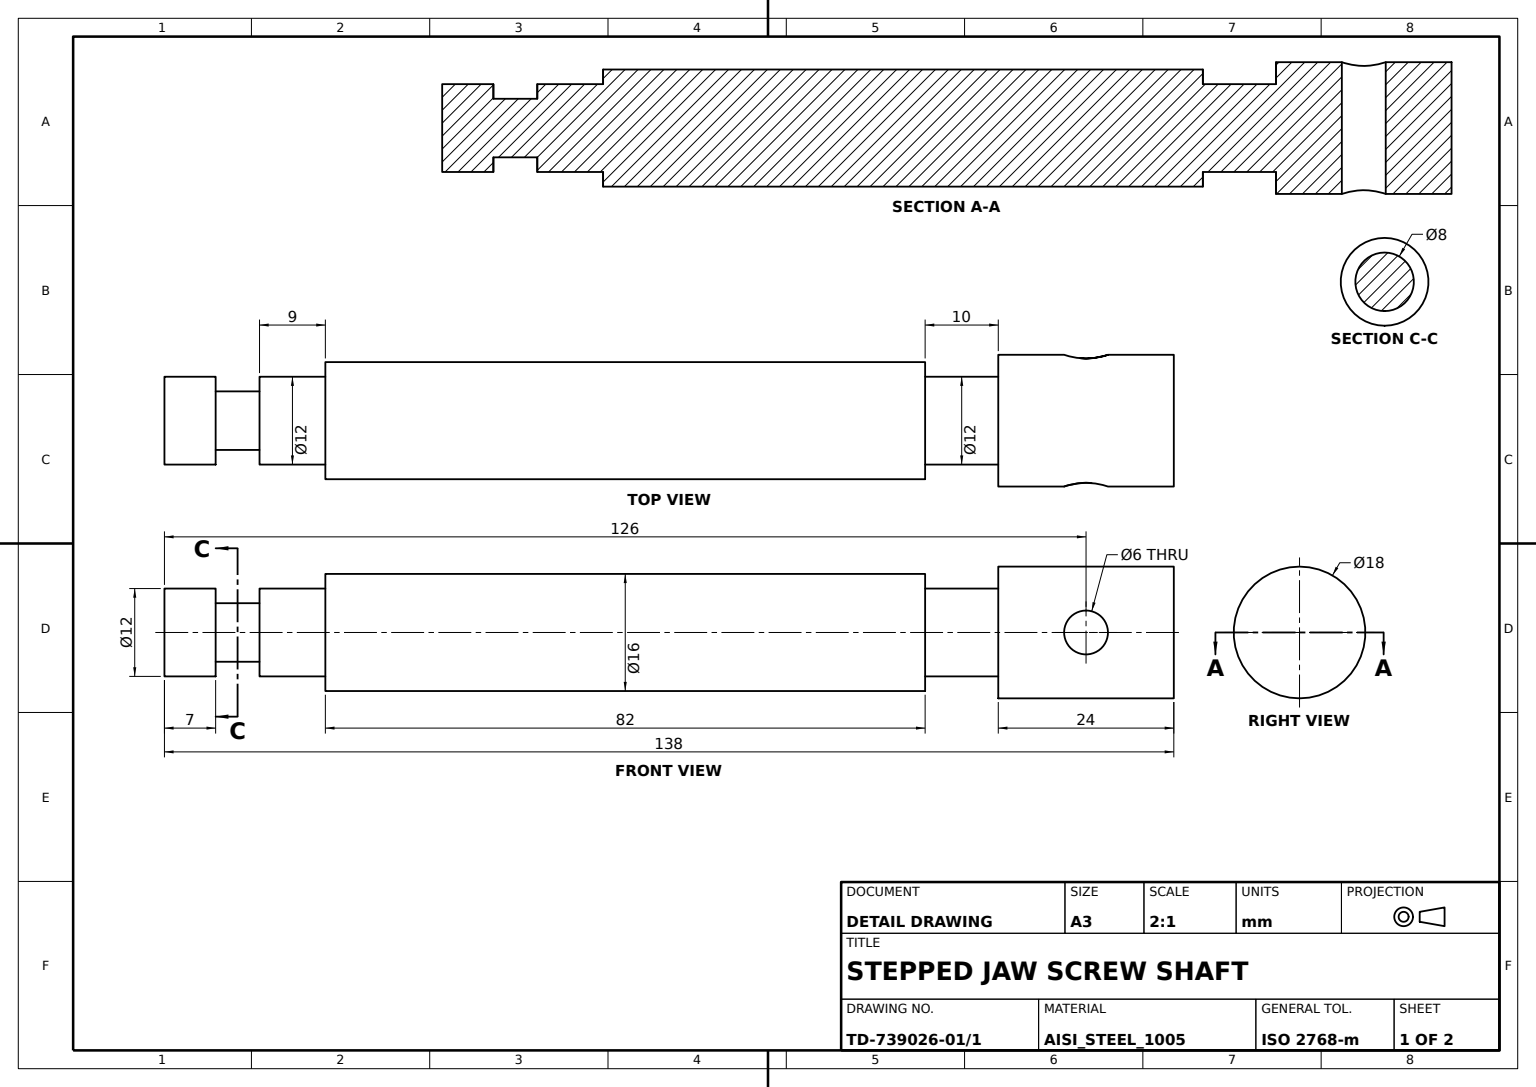
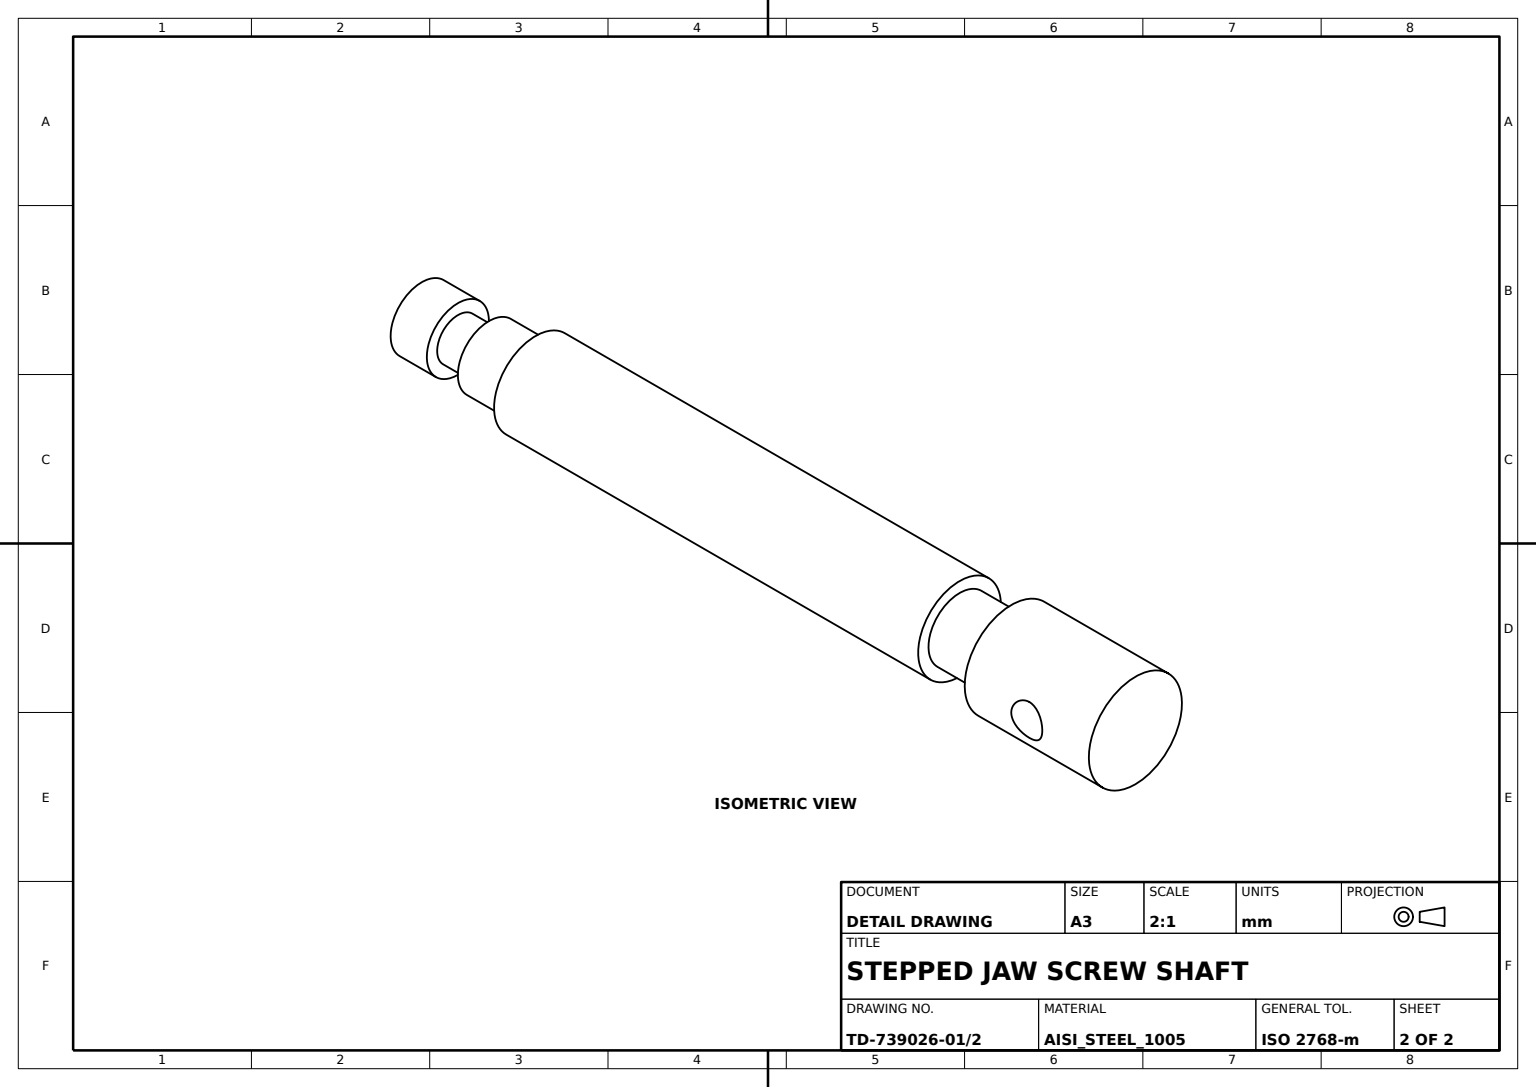
ISO-10303-21;
HEADER;
FILE_DESCRIPTION((''),'2;1');
FILE_NAME('','',(''),(''),'','','');
FILE_SCHEMA(('AUTOMOTIVE_DESIGN'));
ENDSEC;
DATA;
#1=APPLICATION_CONTEXT('');
#2=PRODUCT_CONTEXT('',#1,'mechanical');
#3=PRODUCT('','','',(#2));
#4=PRODUCT_DEFINITION_FORMATION('','',#3);
#5=PRODUCT_DEFINITION_CONTEXT('',#1,'design');
#6=PRODUCT_DEFINITION('','',#4,#5);
#7=PRODUCT_DEFINITION_SHAPE('','',#6);
#8=(LENGTH_UNIT()NAMED_UNIT(*)SI_UNIT(.MILLI.,.METRE.));
#9=(NAMED_UNIT(*)PLANE_ANGLE_UNIT()SI_UNIT($,.RADIAN.));
#10=(NAMED_UNIT(*)SI_UNIT($,.STERADIAN.)SOLID_ANGLE_UNIT());
#11=UNCERTAINTY_MEASURE_WITH_UNIT(LENGTH_MEASURE(0.005),#8,'distance_accuracy_value','');
#12=(GEOMETRIC_REPRESENTATION_CONTEXT(3)GLOBAL_UNCERTAINTY_ASSIGNED_CONTEXT((#11))GLOBAL_UNIT_ASSIGNED_CONTEXT((#8,#9,#10))REPRESENTATION_CONTEXT('',''));
#13=CARTESIAN_POINT('',(0.,48.513563,-9.));
#14=VERTEX_POINT('',#13);
#15=CARTESIAN_POINT('',(0.,48.513563,0.));
#16=DIRECTION('',(0.,-1.,0.));
#17=DIRECTION('',(0.,0.,-1.));
#18=AXIS2_PLACEMENT_3D('',#15,#16,#17);
#19=CIRCLE('',#18,9.);
#20=EDGE_CURVE('',#14,#14,#19,.T.);
#21=ORIENTED_EDGE('',*,*,#20,.T.);
#22=EDGE_LOOP('',(#21));
#23=FACE_BOUND('',#22,.T.);
#24=CARTESIAN_POINT('',(-8.485281,36.513563,3.));
#25=VERTEX_POINT('',#24);
#26=CARTESIAN_POINT('',(-8.75019,34.162799,2.350721));
#27=CARTESIAN_POINT('',(-8.35281,36.513505,3.324938));
#28=CARTESIAN_POINT('',(-8.750258,38.864559,2.349527));
#29=CARTESIAN_POINT('',(-9.124964,39.838536,0.003896));
#30=CARTESIAN_POINT('',(-8.749886,38.862669,-2.353151));
#31=CARTESIAN_POINT('',(-8.352987,36.515667,-3.323633));
#32=CARTESIAN_POINT('',(-8.749854,34.163464,-2.352315));
#33=CARTESIAN_POINT('',(-9.124989,33.188778,0.000128));
#34=B_SPLINE_CURVE_WITH_KNOTS('',3,(#26,#27,#28,#29,#30,#31,#32,#33,#26,#27,#28),.UNSPECIFIED.,.T.,.F.,(1,1,1,1,1,1,1,1,1,1,1,1,1,1,1),(-0.007084493,-0.004722996,-0.002361498,0.,0.002361498,0.004722996,0.007084493,0.009445991,0.011807489,0.014168987,0.016530485,0.018891983,0.02125348,0.023614978,0.025976476),.UNSPECIFIED.);
#35=EDGE_CURVE('',#25,#25,#34,.T.);
#36=ORIENTED_EDGE('',*,*,#35,.F.);
#37=EDGE_LOOP('',(#36));
#38=FACE_BOUND('',#37,.T.);
#39=CARTESIAN_POINT('',(8.485281,36.513563,3.));
#40=VERTEX_POINT('',#39);
#41=CARTESIAN_POINT('',(8.75019,38.864326,2.350721));
#42=CARTESIAN_POINT('',(8.35281,36.513621,3.324938));
#43=CARTESIAN_POINT('',(8.750258,34.162567,2.349527));
#44=CARTESIAN_POINT('',(9.124964,33.188589,0.003896));
#45=CARTESIAN_POINT('',(8.749886,34.164457,-2.353151));
#46=CARTESIAN_POINT('',(8.352987,36.511459,-3.323633));
#47=CARTESIAN_POINT('',(8.749854,38.863662,-2.352315));
#48=CARTESIAN_POINT('',(9.124989,39.838347,0.000128));
#49=B_SPLINE_CURVE_WITH_KNOTS('',3,(#41,#42,#43,#44,#45,#46,#47,#48,#41,#42,#43),.UNSPECIFIED.,.T.,.F.,(1,1,1,1,1,1,1,1,1,1,1,1,1,1,1),(-0.007084493,-0.004722996,-0.002361498,0.,0.002361498,0.004722996,0.007084493,0.009445991,0.011807489,0.014168987,0.016530485,0.018891983,0.02125348,0.023614978,0.025976476),.UNSPECIFIED.);
#50=EDGE_CURVE('',#40,#40,#49,.T.);
#51=ORIENTED_EDGE('',*,*,#50,.F.);
#52=EDGE_LOOP('',(#51));
#53=FACE_BOUND('',#52,.T.);
#54=CARTESIAN_POINT('',(0.,24.513563,-9.));
#55=VERTEX_POINT('',#54);
#56=CARTESIAN_POINT('',(0.,24.513563,0.));
#57=AXIS2_PLACEMENT_3D('',#56,#16,#17);
#58=CIRCLE('',#57,9.);
#59=EDGE_CURVE('',#55,#55,#58,.T.);
#60=ORIENTED_EDGE('',*,*,#59,.F.);
#61=EDGE_LOOP('',(#60));
#62=FACE_BOUND('',#61,.T.);
#63=CARTESIAN_POINT('',(0.,0.,0.));
#64=AXIS2_PLACEMENT_3D('',#63,#16,#17);
#65=CYLINDRICAL_SURFACE('',#64,9.);
#66=ADVANCED_FACE('',(#23,#38,#53,#62),#65,.T.);
#67=CARTESIAN_POINT('',(0.,-67.486437,-8.));
#68=VERTEX_POINT('',#67);
#69=CARTESIAN_POINT('',(0.,-67.486437,0.));
#70=AXIS2_PLACEMENT_3D('',#69,#16,#17);
#71=CIRCLE('',#70,8.);
#72=EDGE_CURVE('',#68,#68,#71,.T.);
#73=ORIENTED_EDGE('',*,*,#72,.T.);
#74=EDGE_LOOP('',(#73));
#75=FACE_BOUND('',#74,.T.);
#76=CARTESIAN_POINT('',(0.,-67.486437,-6.));
#77=VERTEX_POINT('',#76);
#78=CIRCLE('',#70,6.);
#79=EDGE_CURVE('',#77,#77,#78,.T.);
#80=ORIENTED_EDGE('',*,*,#79,.F.);
#81=EDGE_LOOP('',(#80));
#82=FACE_BOUND('',#81,.T.);
#83=CARTESIAN_POINT('',(-8.,-67.486437,0.));
#84=DIRECTION('',(0.,1.,0.));
#85=DIRECTION('',(0.,0.,1.));
#86=AXIS2_PLACEMENT_3D('',#83,#84,#85);
#87=PLANE('',#86);
#88=ADVANCED_FACE('',(#75,#82),#87,.F.);
#89=CARTESIAN_POINT('',(0.,-82.486437,-4.));
#90=VERTEX_POINT('',#89);
#91=CARTESIAN_POINT('',(0.,-82.486437,0.));
#92=AXIS2_PLACEMENT_3D('',#91,#16,#17);
#93=CIRCLE('',#92,4.);
#94=EDGE_CURVE('',#90,#90,#93,.T.);
#95=ORIENTED_EDGE('',*,*,#94,.T.);
#96=EDGE_LOOP('',(#95));
#97=FACE_BOUND('',#96,.T.);
#98=CARTESIAN_POINT('',(0.,-82.486437,-6.));
#99=VERTEX_POINT('',#98);
#100=CIRCLE('',#92,6.);
#101=EDGE_CURVE('',#99,#99,#100,.T.);
#102=ORIENTED_EDGE('',*,*,#101,.F.);
#103=EDGE_LOOP('',(#102));
#104=FACE_BOUND('',#103,.T.);
#105=CARTESIAN_POINT('',(-4.,-82.486437,0.));
#106=AXIS2_PLACEMENT_3D('',#105,#16,#17);
#107=PLANE('',#106);
#108=ADVANCED_FACE('',(#97,#104),#107,.F.);
#109=CARTESIAN_POINT('',(0.,-76.486437,-6.));
#110=VERTEX_POINT('',#109);
#111=CARTESIAN_POINT('',(0.,-76.486437,0.));
#112=AXIS2_PLACEMENT_3D('',#111,#16,#17);
#113=CIRCLE('',#112,6.);
#114=EDGE_CURVE('',#110,#110,#113,.T.);
#115=ORIENTED_EDGE('',*,*,#114,.F.);
#116=EDGE_LOOP('',(#115));
#117=FACE_BOUND('',#116,.T.);
#118=ORIENTED_EDGE('',*,*,#79,.T.);
#119=EDGE_LOOP('',(#118));
#120=FACE_BOUND('',#119,.T.);
#121=CYLINDRICAL_SURFACE('',#64,6.);
#122=ADVANCED_FACE('',(#117,#120),#121,.T.);
#123=CARTESIAN_POINT('',(0.,14.513563,-6.));
#124=VERTEX_POINT('',#123);
#125=CARTESIAN_POINT('',(0.,14.513563,0.));
#126=AXIS2_PLACEMENT_3D('',#125,#16,#17);
#127=CIRCLE('',#126,6.);
#128=EDGE_CURVE('',#124,#124,#127,.T.);
#129=ORIENTED_EDGE('',*,*,#128,.F.);
#130=EDGE_LOOP('',(#129));
#131=FACE_BOUND('',#130,.T.);
#132=CARTESIAN_POINT('',(0.,24.513563,-6.));
#133=VERTEX_POINT('',#132);
#134=CIRCLE('',#57,6.);
#135=EDGE_CURVE('',#133,#133,#134,.T.);
#136=ORIENTED_EDGE('',*,*,#135,.T.);
#137=EDGE_LOOP('',(#136));
#138=FACE_BOUND('',#137,.T.);
#139=ADVANCED_FACE('',(#131,#138),#121,.T.);
#140=ORIENTED_EDGE('',*,*,#35,.T.);
#141=EDGE_LOOP('',(#140));
#142=FACE_BOUND('',#141,.T.);
#143=ORIENTED_EDGE('',*,*,#50,.T.);
#144=EDGE_LOOP('',(#143));
#145=FACE_BOUND('',#144,.T.);
#146=CARTESIAN_POINT('',(12.,36.513563,0.));
#147=DIRECTION('',(-1.,0.,0.));
#148=AXIS2_PLACEMENT_3D('',#146,#147,#85);
#149=CYLINDRICAL_SURFACE('',#148,3.);
#150=ADVANCED_FACE('',(#142,#145),#149,.F.);
#151=ORIENTED_EDGE('',*,*,#59,.T.);
#152=EDGE_LOOP('',(#151));
#153=FACE_BOUND('',#152,.T.);
#154=ORIENTED_EDGE('',*,*,#135,.F.);
#155=EDGE_LOOP('',(#154));
#156=FACE_BOUND('',#155,.T.);
#157=CARTESIAN_POINT('',(-9.,24.513563,0.));
#158=AXIS2_PLACEMENT_3D('',#157,#84,#85);
#159=PLANE('',#158);
#160=ADVANCED_FACE('',(#153,#156),#159,.F.);
#161=CARTESIAN_POINT('',(0.,-89.486437,-6.));
#162=VERTEX_POINT('',#161);
#163=CARTESIAN_POINT('',(0.,-89.486437,0.));
#164=AXIS2_PLACEMENT_3D('',#163,#16,#17);
#165=CIRCLE('',#164,6.);
#166=EDGE_CURVE('',#162,#162,#165,.T.);
#167=ORIENTED_EDGE('',*,*,#166,.F.);
#168=EDGE_LOOP('',(#167));
#169=FACE_BOUND('',#168,.T.);
#170=ORIENTED_EDGE('',*,*,#101,.T.);
#171=EDGE_LOOP('',(#170));
#172=FACE_BOUND('',#171,.T.);
#173=ADVANCED_FACE('',(#169,#172),#121,.T.);
#174=ORIENTED_EDGE('',*,*,#72,.F.);
#175=EDGE_LOOP('',(#174));
#176=FACE_BOUND('',#175,.T.);
#177=CARTESIAN_POINT('',(0.,14.513563,-8.));
#178=VERTEX_POINT('',#177);
#179=CIRCLE('',#126,8.);
#180=EDGE_CURVE('',#178,#178,#179,.T.);
#181=ORIENTED_EDGE('',*,*,#180,.T.);
#182=EDGE_LOOP('',(#181));
#183=FACE_BOUND('',#182,.T.);
#184=CYLINDRICAL_SURFACE('',#64,8.);
#185=ADVANCED_FACE('',(#176,#183),#184,.T.);
#186=ORIENTED_EDGE('',*,*,#166,.T.);
#187=EDGE_LOOP('',(#186));
#188=FACE_BOUND('',#187,.T.);
#189=CARTESIAN_POINT('',(-6.,-89.486437,0.));
#190=AXIS2_PLACEMENT_3D('',#189,#84,#85);
#191=PLANE('',#190);
#192=ADVANCED_FACE('',(#188),#191,.F.);
#193=ORIENTED_EDGE('',*,*,#114,.T.);
#194=EDGE_LOOP('',(#193));
#195=FACE_BOUND('',#194,.T.);
#196=CARTESIAN_POINT('',(0.,-76.486437,-4.));
#197=VERTEX_POINT('',#196);
#198=CIRCLE('',#112,4.);
#199=EDGE_CURVE('',#197,#197,#198,.T.);
#200=ORIENTED_EDGE('',*,*,#199,.F.);
#201=EDGE_LOOP('',(#200));
#202=FACE_BOUND('',#201,.T.);
#203=CARTESIAN_POINT('',(-6.,-76.486437,0.));
#204=AXIS2_PLACEMENT_3D('',#203,#84,#85);
#205=PLANE('',#204);
#206=ADVANCED_FACE('',(#195,#202),#205,.F.);
#207=ORIENTED_EDGE('',*,*,#128,.T.);
#208=EDGE_LOOP('',(#207));
#209=FACE_BOUND('',#208,.T.);
#210=ORIENTED_EDGE('',*,*,#180,.F.);
#211=EDGE_LOOP('',(#210));
#212=FACE_BOUND('',#211,.T.);
#213=CARTESIAN_POINT('',(-6.,14.513563,0.));
#214=AXIS2_PLACEMENT_3D('',#213,#16,#17);
#215=PLANE('',#214);
#216=ADVANCED_FACE('',(#209,#212),#215,.F.);
#217=ORIENTED_EDGE('',*,*,#199,.T.);
#218=EDGE_LOOP('',(#217));
#219=FACE_BOUND('',#218,.T.);
#220=ORIENTED_EDGE('',*,*,#94,.F.);
#221=EDGE_LOOP('',(#220));
#222=FACE_BOUND('',#221,.T.);
#223=CYLINDRICAL_SURFACE('',#64,4.);
#224=ADVANCED_FACE('',(#219,#222),#223,.T.);
#225=ORIENTED_EDGE('',*,*,#20,.F.);
#226=EDGE_LOOP('',(#225));
#227=FACE_BOUND('',#226,.T.);
#228=PLANE('',#18);
#229=ADVANCED_FACE('',(#227),#228,.F.);
#230=CLOSED_SHELL('',(#66,#88,#108,#122,#139,#150,#160,#173,#185,#192,#206,#216,#224,#229));
#231=MANIFOLD_SOLID_BREP('',#230);
#232=ADVANCED_BREP_SHAPE_REPRESENTATION('',(#231),#12);
#233=SHAPE_DEFINITION_REPRESENTATION(#7,#232);
ENDSEC;
END-ISO-10303-21;
